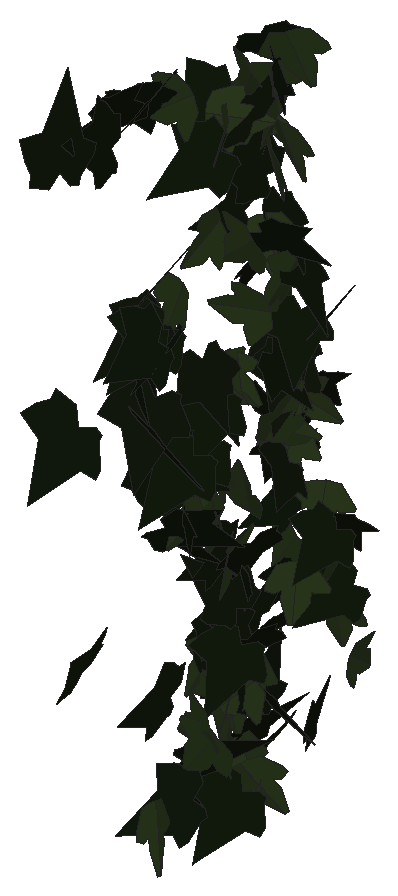
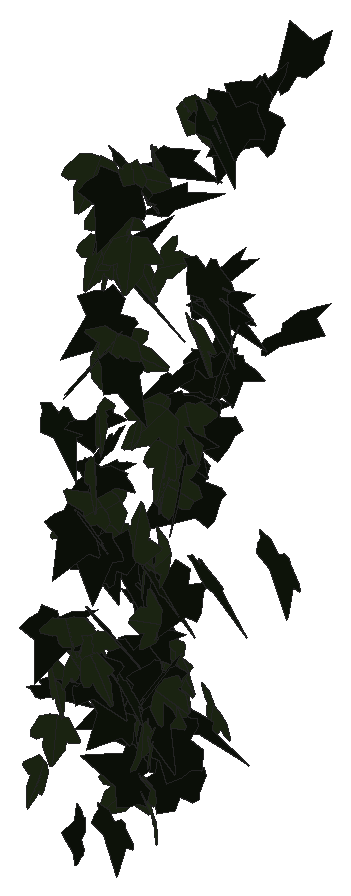
# SketchUp Ruby script. Lengths in inches.
U = 1.inch
M = Sketchup.active_model
def pt(a) = Geom::Point3d.new(a.map { |v| v * U })
def face(e, loops, mat)
  f = e.add_face(loops[0].map { |a| pt(a) })
  loops[1..].each { |l| e.add_face(l.map { |a| pt(a) }).erase! }
  f.material = f.back_material = mat if mat
  f
end
# faces: each face lists its corners as indices into pts; further lists are holes
def faces(e, pts, list, mat = nil) = list.each { |f| face(e, (f[0].is_a?(Array) ? f : [f]).map { |l| l.map { |i| pts[i] } }, mat) }
# xy, xz, yz: faces in a plane at the given z, y or x. An outline is a flat list of corners, or four numbers for a rectangle; further outlines are holes
def ring(l) = l.size == 4 ? [[l[0], l[1]], [l[2], l[1]], [l[2], l[3]], [l[0], l[3]]] : l.each_slice(2).to_a
def flat(e, list, mat, &to3) = list.each { |f| face(e, (f[0].is_a?(Array) ? f : [f]).map { |l| ring(l).map { |u, v| to3.(u, v) } }, mat) }
def xy(e, z, list, mat = nil) = flat(e, list, mat) { |x, y| [x, y, z] }
def xz(e, y, list, mat = nil) = flat(e, list, mat) { |x, z| [x, y, z] }
def yz(e, x, list, mat = nil) = flat(e, list, mat) { |y, z| [x, y, z] }
def lines(e, pts, list) = list.each { |a, b| e.add_line(pt(pts[a]), pt(pts[b])) }
# prism: a flat outline (further loops are holes) pulled along v
def prism(e, loops, v, mat = nil)
  f = face(e, loops, mat); d = Geom::Vector3d.new(v.map { |x| x * U })
  f.pushpull(f.normal.samedirection?(d) ? d.length : -d.length)
end
def box(e, o, s, mat = nil) = prism(e, [[o, [o[0] + s[0], o[1], o[2]], [o[0] + s[0], o[1] + s[1], o[2]], [o[0], o[1] + s[1], o[2]]]], [0, 0, s[2]], mat)
def at(x, y, z, deg = 0) = Geom::Transformation.translation(pt([x, y, z])) * Geom::Transformation.rotation(ORIGIN, Z_AXIS, deg.degrees)
def axes(o, x, y, z) = Geom::Transformation.new([*x, 0, *y, 0, *z, 0, *pt(o).to_a, 1])
def part(name) = M.definitions.add(name)
# library, detail: a bought-in or finely detailed component or shape, given as its bounding box
def library(name, o, s) = part(name).tap { |d| box(d.entities, o, s) }
def detail(e, o, s) = box(e.add_group.entities, o, s)
def put(e, d, t, mat = nil) = e.add_instance(d, t).tap { |i| i.material = mat if mat }
def group(e, t, mat = nil) = e.add_group.tap { |g| g.transformation = t; g.material = mat if mat }.entities
root = M.entities
M.materials.add("efeu1").color = [18, 25, 13]
M.materials.add("efeu2").color = [43, 57, 29]
c1 = part("ivyleaf_10")
p = [[0,0.5,-0.03],[-0.0625,2.02,-0.43],[-0.19,2.01,-0.46],[-0.54,1.05,-0.29],[-0.52,0.625,-0.18],[-0.83,0.76,-0.28],
  [-1.16,0.64,-0.33],[-1.15,0.33,-0.24],[-0.77,-0.39,0.02],[-0.3,-0.51,0.16],[0.04,-0.48,0.23],[-0.02,2.01,-0.4375],
  [-0.06,2.01,-0.43],[0.04,-0.49,0.23],[0.67,-0.49,0.14],[1.38,0.36,-0.2],[1.375,0.51,-0.24],[0.81,0.65,-0.19],
  [0.62,0.59,-0.15],[0.6,1.09,-0.28],[0.5,1.23,-0.31]]
faces(c1.entities,p,[[0,1,2,3,4,5,6,7,8,9,10],[11,12,0,13,14,15,16,17,18,19,20]],"efeu2")
c2 = part("ivyleaf_9")
p = [[1.54,2.16,1.25],[1.36,2.04,1.19],[-0.21,0.99,0.68],[-0.71,1.11,0.82],[-0.85,0.86,0.67],[-0.8,0.17,0.21],
  [-0.9,-0.01,0.1],[-0.67,-0.16,-0.02],[-0.08,-0.08,-0.05],[-0.03,-0.6,-0.4],[0.65,-0.88,-0.66],[0.83,-0.6,-0.49],
  [1.29,-0.42,-0.43],[1.8125,-0.07,-0.26],[1.21,0.44,0.15]]
faces(c2.entities,p,[[0,1,2,3,4,5,6,7,8,9,10,11,12,13,14]],"efeu1")
put(root,c1,axes([501.72,128.93,272.02],[-0.78096,-0.6795,-0.10689],[0.05982,0.09109,-1.03155],[0.73979,-0.72468,-0.02943]))
put(root,c2,axes([502.21,117.86,251.28],[-0.29268,0.97314,0.57352],[-0.16847,0.52899,-1.05055],[-1.19621,-0.3126,0.00763]))
put(root,c1,axes([501.68,126.66,248.28],[-0.09087,-0.69391,0.75827],[0.12672,-0.76299,-0.68304],[1.02001,0.03297,0.15241]))
put(root,c2,axes([502.08,129.67,242.97],[-0.12007,0.83731,0.36079],[-0.10194,0.33692,-0.87717],[-0.97351,-0.13855,0.04735]))
put(root,c2,axes([502.22,126.26,272.94],[-0.68822,-0.27679,0.78402],[-0.61332,-0.52516,-0.69977],[0.61326,-0.83583,0.18003]))
put(root,c2,axes([501.44,125.36,253.35],[1.1608,0.21664,-0.27086],[-0.31452,0.14824,-1.12166],[-0.18691,1.09594,0.20526]))
put(root,c2,axes([502.32,126.64,247.25],[0.30514,0.22931,-0.9611],[-0.97083,-0.2536,-0.35127],[-0.33906,0.9325,0.14081]))
put(root,c1,axes([501.35,127.875,242.7],[-0.3025,0.00297,-0.93347],[0.46003,-0.82719,-0.14109],[-0.85327,-0.44702,0.25487]))
put(root,c1,axes([502.36,130.77,251.37],[-0.76072,0.09915,0.57402],[-0.60564,-0.12345,-0.7212],[-0.00074,-0.8863,0.16467]))
put(root,c2,axes([502.51,130.46,253.66],[-0.94565,0.41354,0.12892],[-0.12249,0.04165,-1.03206],[-0.4155,-0.95349,0.01083]))
put(root,c2,axes([501.66,119.5,274.81],[0.56458,0.79306,0.80806],[0.4864,0.6335,-0.9876],[-1.09598,0.68968,-0.02204]))
put(root,c1,axes([502.04,126.88,251.94],[0.27281,-0.49023,0.87991],[-0.24877,0.81942,0.56531],[-1.02634,-0.32893,0.09686]))
put(root,c2,axes([501.3,130.58,256.63],[-0.01634,-0.24646,1.0091],[0.78003,-0.66939,-0.15086],[0.68598,0.75529,0.19558]))
put(root,c2,axes([502.65,128.3125,249.42],[-0.33388,0.68229,0.61589],[-0.33221,0.50902,-0.77692],[-0.91743,-0.43263,0.05719]))
put(root,c2,axes([502.13,121.05,275.42],[0.6466,0.91322,-0.19977],[-0.12195,-0.15565,-1.13562],[-1.00046,0.60919,0.00931]))
put(root,c2,axes([501.7,126.62,249.36],[0.51989,-0.80612,-0.39129],[-0.1805,0.34889,-0.9586],[0.8777,0.54925,0.03463]))
put(root,c2,axes([502.28,130.8,257.76],[0.64094,0.53886,-0.51639],[-0.41388,-0.31635,-0.83341],[-0.6745,0.70616,0.02069]))
put(root,c2,axes([501.85,126.65,249.34],[0.09255,-0.43655,-1.00064],[-0.15444,0.95164,-0.4623],[1.13058,0.16573,0.01876]))
put(root,c1,axes([502.3,127.27,245.49],[-0.11036,0.91847,-0.43534],[-0.04461,0.41658,0.96109],[1.0892,0.11013,-0.00474]))
put(root,c1,axes([502.49,130.73,261.33],[-0.69678,0.59318,0.37254],[-0.44044,0.07068,-0.8856],[-0.60506,-0.73455,0.21563]))
put(root,c1,axes([502.22,123.66,265.4],[0.98062,-0.57679,-0.12791],[-0.11605,0.06021,-1.11869],[0.62627,0.91429,-0.00702]))
put(root,c2,axes([502.7,121.59,275.1875],[-0.37673,1.046,0.02923],[-0.01204,0.0259,-1.14673],[-1.13002,-0.34899,0.00248]))
put(root,c2,axes([502.25,129.01,248.27],[0.40688,0.66465,0.56286],[0.12667,0.54564,-0.78181],[-0.91699,0.37029,0.14175]))
put(root,c2,axes([502.9375,125.71,253.41],[-0.87145,0.63548,0.10554],[-0.08486,0.06424,-1.06818],[-0.68981,-0.81072,-0.00192]))
put(root,c1,axes([502.69,125.27,254.37],[0.29546,-0.21031,0.99562],[-0.61259,0.77661,0.34601],[-0.8633,-0.62305,0.09521]))
put(root,c2,axes([502.68,121.54,261.6875],[0.13142,-0.8987,0.78595],[0.02404,0.7614,0.93794],[-1.26792,-0.07871,0.09924]))
put(root,c2,axes([502.39,128.78,274.71],[0.60354,0.84814,-0.01727],[-0.00637,-0.016,-1.05631],[-0.91614,0.55885,-0.00403]))
put(root,c2,axes([502.75,131.06,258.8125],[-0.94972,0.23126,-0.22964],[0.23788,-0.03027,-0.94525],[-0.25032,-0.90616,-0.02703]))
put(root,c2,axes([502.91,121.4,265.32],[-1.1589,-0.1407,0.02537],[-0.02545,-0.00795,-1.12552],[0.15211,-1.0733,0.00501]))
put(root,c2,axes([502.44,117.17,262.4],[-0.51227,-1.08029,0.53888],[-0.21565,-0.47821,-1.227],[1.27589,-0.51457,0.00897]))
put(root,c2,axes([502.85,128.32,265.54],[-0.40997,0.86111,-0.42499],[0.15795,-0.38203,-0.97852],[-1.01722,-0.40638,0.01934]))
put(root,c2,axes([503.04,121.88,267.28],[-0.4821,1.07553,-0.04386],[-0.00007,-0.04568,-1.21093],[-1.16246,-0.44604,0.01826]))
put(root,c2,axes([502.82,130.18,250.71],[-0.08384,0.5825,-0.74236],[0.0297,-0.71455,-0.60954],[-0.99458,-0.07044,0.04437]))
put(root,c2,axes([502.61,131.37,242.76],[0.04801,-0.00313,0.90204],[0.2179,0.8447,-0.00759],[-0.91104,0.20187,0.04572]))
put(root,c1,axes([502.43,128.02,273.21],[-0.67854,0.77843,-0.17211],[0.10682,-0.13283,-1.04034],[-0.85283,-0.63599,0.00663]))
put(root,c2,axes([503.26,126.41,268.26],[-0.84821,0.56452,0.24472],[-0.24715,0.08392,-1.00373],[-0.61255,-0.81556,0.06611]))
put(root,c1,axes([502.58,126.25,247.27],[-1.09261,-0.41527,-0.15628],[0.1886,-0.03118,-1.13309],[0.43807,-1.0223,0.09804]))
put(root,c1,axes([502.38,128.18,271.125],[0.39667,0.94718,0.03913],[0.01781,0.03395,-1.05653],[-1.02361,0.36764,-0.00322]))
put(root,c2,axes([502.24,124.85,242.35],[0.77152,0.6545,0.4461],[-0.33554,-0.29584,1.00759],[0.77568,-0.77897,-0.00785]))
put(root,c1,axes([502.3125,126.85,245.67],[0.00305,0.02034,-1.06011],[0.27283,-0.98757,-0.01977],[-1.06677,-0.25251,-0.00809]))
put(root,c2,axes([502.74,118.9,274.18],[-0.1507,-0.14254,1.17854],[-0.49712,-1.0378,-0.19471],[1.1289,-0.47604,0.07159]))
put(root,c2,axes([502.86,115.69,274.72],[-0.51525,-0.72738,0.993],[0.66598,0.73298,0.90117],[-1.11218,0.7759,0.07959]))
put(root,c1,axes([502.89,123.36,260.6],[-0.1271,-1.05619,0.07366],[-0.00448,-0.0708,-1.10523],[1.14324,-0.1177,0.00385]))
put(root,c1,axes([502.875,128.75,273.29],[-0.82233,-0.65785,-0.09973],[0.0826,0.05815,-1.04647],[0.71322,-0.76523,0.00621]))
put(root,c2,axes([502.4,127.52,244.3],[0.0977,0.92451,-0.40102],[0.0265,0.38501,0.966],[1.08151,-0.09295,0.01255]))
put(root,c2,axes([503.1,129.39,256.82],[0.09782,0.81046,-0.50619],[-0.10808,-0.47799,-0.84711],[-1.01528,0.12897,0.04141]))
put(root,c2,axes([502.8,130.98,258.36],[0.52486,0.77685,0.19284],[0.11522,0.15197,-0.95294],[-0.85484,0.49746,-0.01003]))
put(root,c2,axes([503.72,125.37,251.48],[-0.20153,0.3281,0.95737],[-0.90014,0.43593,-0.33729],[-0.55111,-0.83199,0.20081]))
put(root,c2,axes([502.4,124.15,244.7],[0.17546,0.77238,-0.84602],[0.17513,0.79716,0.82084],[1.19876,-0.22951,0.00391]))
put(root,c1,axes([503.5,126.72,274.12],[-0.88327,0.27039,0.66885],[-0.65869,0.20404,-0.89583],[-0.36583,-1.02022,-0.0019]))
put(root,c2,axes([502.47,129.93,266.83],[0.40664,-0.8982,0.01344],[0.01251,-0.00916,-1.01286],[0.97008,0.37663,0.00743]))
put(root,c2,axes([502.61,129.93,260.92],[-0.52396,-0.62003,-0.67499],[0.58726,0.36983,-0.79557],[0.70368,-0.77031,0.16135]))
put(root,c1,axes([502.85,129.64,263.35],[0.35109,-0.97546,0.2369],[0.34439,-0.11869,-0.99911],[0.94289,0.40657,0.27671]))
put(root,c1,axes([503.08,131.4,251.75],[-0.16641,0.71349,-0.57631],[-0.12014,-0.57285,-0.73492],[-0.96826,-0.05155,0.19023]))
put(root,c1,axes([503.21,126.71,255.28],[-1.05007,0.19697,0.03456],[0.03125,-0.02454,1.03155],[0.21346,0.97255,0.01902]))
put(root,c1,axes([503.7,122.12,275.28],[0.73402,-0.19724,-0.85795],[-0.82942,0.30568,-0.73403],[0.38889,1.02422,0.05385]))
put(root,c1,axes([502.56,127.27,243.9],[0.84539,0.00314,0.6131],[0.63661,-0.01972,-0.81388],[0.0101,0.97973,-0.01835]))
put(root,c2,axes([503.76,125.78,253.02],[0.10141,0.08594,-1.01237],[-1.05528,-0.00627,-0.0986],[-0.01568,0.97793,0.08833]))
put(root,c2,axes([503.41,121.21,265.31],[-0.83727,-0.71043,0.23086],[-0.17764,-0.14907,-1.0936],[0.78398,-0.79251,-0.00125]))
put(root,c1,axes([502.87,125.61,261.54],[-0.69758,-0.41775,-0.69608],[0.68153,0.19729,-0.80141],[0.44109,-0.96551,0.13741]))
put(root,c1,axes([503.17,131.54,253.52],[0.82028,0.49041,-0.09924],[-0.07878,-0.06292,-0.94015],[-0.5338,0.7629,-0.01375]))
put(root,c2,axes([503.52,128.14,274.08],[0.51,-0.10683,-0.93608],[-0.87215,0.4113,-0.4914],[0.44454,0.9295,0.10986]))
put(root,c1,axes([503.8,125.98,247.63],[0.81202,-0.01274,-0.67385],[-0.69618,0.0875,-0.77973],[0.07208,0.98867,0.06033]))
put(root,c2,axes([503.21,129.58,260.22],[-0.33939,-1.01454,0.0589],[0.01675,-0.06767,-1.06916],[1.01611,-0.33775,0.03729]))
put(root,c2,axes([503.32,120.91,262.28],[-0.97572,-0.66022,-0.48489],[0.40607,0.27571,-1.16374],[0.77272,-0.97856,-0.00073]))
put(root,c2,axes([504.18,122.05,244.44],[-1.20392,0.17857,0.30785],[-0.31574,0.04639,-1.17412],[-0.19926,-1.15244,0.00044]))
put(root,c1,axes([503.33,124.94,261.65],[-0.09444,0.79519,0.72775],[-0.05462,0.72607,-0.80044],[-1.07655,-0.10659,-0.02323]))
put(root,c2,axes([503.82,127.08,269.84],[-0.19751,0.07639,1.06889],[-0.8386,-0.69658,-0.08985],[0.73189,-0.77753,0.1855]))
put(root,c1,axes([503.02,128.29,266.61],[0.9831,0.319,0.35597],[0.34955,0.11136,-1.00313],[-0.3649,0.9661,-0.00191]))
put(root,c1,axes([503.41,129.23,257.11],[0.94753,0.33113,-0.15832],[-0.15166,-0.05904,-0.97524],[-0.36321,0.88849,-0.0058]))
put(root,c1,axes([503.4,124.88,246.18],[-0.54743,0.8672,-0.0376],[0.01982,-0.03116,-1.04465],[-0.93718,-0.50721,-0.00013]))
put(root,c1,axes([503.62,131.95,248.43],[-0.93335,-0.19237,0.04711],[-0.0445,-0.02337,-0.92067],[0.20875,-0.86508,0.0144]))
put(root,c2,axes([503.03,121.25,259.45],[0.25769,-0.09773,-1.22069],[-0.08279,1.19376,-0.11957],[1.26933,0.0977,0.24002]))
put(root,c2,axes([503.75,126.2,249.54],[0.12437,0.94431,-0.26799],[-0.03234,-0.25594,-0.98936],[-1.05665,0.11898,-0.00127]))
put(root,c2,axes([503.77,123.47,259.38],[-1.04224,-0.56009,-0.15295],[0.11804,0.10452,-1.15985],[0.61416,-0.97057,-0.03664]))
put(root,c2,axes([504.22,120.2,264.83],[-0.51275,1.03756,0.20388],[-0.12785,0.16129,-1.18594],[-1.13321,-0.48767,0.04155]))
put(root,c1,axes([503.6,124.32,268.47],[0.10217,0.3736,-1.04423],[-0.21587,-0.98412,-0.40042],[-1.13671,0.22047,-0.01781]))
put(root,c1,axes([503.71,124.08,258.64],[-1.0243,0.45629,0.11146],[-0.10397,0.04711,-1.09458],[-0.49541,-0.9533,-0.00074]))
put(root,c1,axes([503.8125,123.51,256.77],[-0.26663,-0.61891,0.87573],[-0.07577,-0.85346,-0.67378],[1.12609,-0.20397,0.16202]))
put(root,c1,axes([503.73,131.78,250.82],[0.25255,-0.86865,-0.07681],[-0.03132,0.06868,-0.9355],[0.94101,0.23542,-0.01052]))
put(root,c2,axes([503.86,122.37,257.39],[0.42845,-0.25651,-1.02312],[-0.92131,0.49049,-0.49077],[0.59732,0.94053,-0.0231]))
put(root,c1,axes([503.1,129.9375,258.5625],[0.54841,0.20725,0.88486],[0.55429,0.74273,-0.51749],[-0.72021,0.72944,0.27552]))
put(root,c1,axes([503.53,125.49,253.83],[-0.26729,0.59919,-0.80041],[0.06646,-0.78284,-0.65443],[-1.0513,-0.20183,0.16213]))
put(root,c1,axes([503.24,128.3125,271.52],[0.00388,0.0197,1.06145],[0.69067,-0.79557,0.01363],[0.85932,0.63934,-0.01574]))
put(root,c1,axes([503.99,122.37,258.03],[-0.13601,0.21203,1.10607],[-0.53144,0.94294,-0.25611],[-1.0437,-0.50776,-0.01373]))
put(root,c1,axes([504.5,125.78,264.59],[0.21446,0.04379,-1.04068],[-1.07198,0.14535,-0.19823],[0.145,1.00976,0.07367]))
put(root,c1,axes([503.38,126.79,243.33],[-0.85887,-0.24834,-0.6251],[0.62949,0.14897,-0.86604],[0.31154,-0.98565,0.02661]))
put(root,c1,axes([503.39,128.3,257.99],[-0.35284,-0.33743,-0.89319],[0.64467,0.61749,-0.48846],[0.75997,-0.68047,-0.00034]))
put(root,c1,axes([504.57,122.55,247.47],[-0.45503,0.04623,0.99267],[-1.0181,0.15088,-0.44036],[-0.16917,-1.03238,-0.01991]))
put(root,c2,axes([503.39,123.95,262.68],[0.31021,-0.95965,-0.5692],[-0.14841,0.53007,-1.04162],[1.18386,0.31791,0.01857]))
put(root,c2,axes([503.57,128.0625,261.23],[0.52717,-0.52357,-0.69228],[-0.39854,0.56004,-0.73954],[0.82324,0.60639,0.08529]))
put(root,c1,axes([503.68,127.91,258.1],[-0.05884,-0.91706,0.48775],[0.02776,0.46829,0.95542],[-1.11208,0.06021,-0.00196]))
put(root,c1,axes([503.78,128.56,270.98],[-1.016,0.35149,-0.14254],[0.14658,-0.02825,-1.0442],[-0.38017,-0.95025,-0.02168]))
put(root,c2,axes([503.4,121.78,256.33],[0.92733,0.68329,0.54176],[0.43496,0.33048,-1.14121],[-0.8197,0.94838,0.00734]))
put(root,c2,axes([503.82,126.8,246.65],[-0.17014,-0.50171,0.8615],[0.62665,0.62305,0.50721],[-0.83742,0.56817,0.20452]))
put(root,c1,axes([504.11,132.37,246.15],[0.06777,0.49284,0.7562],[-0.40657,0.67372,-0.44113],[-0.85714,-0.2806,0.26903]))
put(root,c2,axes([503.95,124.02,261.1875],[-0.62245,-0.8518,-0.01068],[0.00758,0.00766,-1.06959],[0.91998,-0.57638,0.00158]))
put(root,c1,axes([503.64,126.56,248.24],[1.01168,-0.09174,0.29659],[0.31076,0.01503,-0.97794],[0.09003,0.97907,0.0428]))
put(root,c2,axes([503.8125,129.36,262.65],[-0.36836,-0.91749,-0.19117],[0.06311,0.17438,-1.01797],[1.00861,-0.34599,-0.00612]))
put(root,c1,axes([504.34,123.21,257.6],[-0.60158,0.58799,0.65844],[-0.48853,0.44336,-0.84211],[-0.79507,-0.71731,0.01923]))
put(root,c2,axes([504.1,125.23,249.81],[-0.71305,-0.78739,0.01187],[-0.00372,-0.012,-1.06865],[0.85046,-0.66022,0.00527]))
put(root,c2,axes([504.79,125.12,273.375],[-0.38637,0.82498,0.63675],[-0.49344,0.45333,-0.88675],[-0.9179,-0.59095,0.20867]))
put(root,c2,axes([504.08,120.09,265.52],[-0.35993,-0.69205,0.90842],[-0.34582,-0.8138,-0.7976],[1.15281,-0.46019,0.04436]))
put(root,c1,axes([504.21,127.2,270.71],[-0.8018,0.70772,0.23513],[-0.19347,0.13602,-1.06916],[-0.72022,-0.82442,0.02544]))
put(root,c2,axes([504.38,125.55,254.27],[-0.04767,0.95541,-0.30981],[0.04555,-0.29614,-0.99429],[-1.07988,-0.05467,-0.02827]))
put(root,c1,axes([503.26,125.11,273.15],[0.10485,-0.30463,-1.00732],[1.09243,0.11356,0.0683],[0.09529,-0.96678,0.32543]))
put(root,c1,axes([504.03,128.58,275.12],[-0.96406,-0.45281,-0.30173],[0.28999,0.09185,-1.06441],[0.46042,-1.00599,0.03863]))
put(root,c1,axes([503.98,128.86,251.35],[0.81974,0.55403,-0.04832],[-0.03649,-0.03253,-0.97728],[-0.59935,0.75974,-0.0066]))
put(root,c2,axes([504.53,131.5,249.9],[-0.86119,-0.34755,0.26642],[-0.22773,-0.15601,-0.90274],[0.40691,-0.82288,0.05863]))
put(root,c1,axes([503.61,120.5625,244.21],[0.8662,-0.32864,0.67045],[0.64305,-0.24713,-0.90142],[0.44408,0.99889,-0.00243]))
put(root,c2,axes([503.27,120.48,261.26],[0.89727,-0.57473,0.48007],[0.41306,-0.2585,-1.05062],[0.68059,0.9146,0.00473]))
put(root,c2,axes([504.11,131.04,252.93],[0.77889,0.54112,-0.19509],[-0.23216,-0.02384,-0.93099],[-0.57331,0.74481,0.11194]))
put(root,c1,axes([504.81,122.59,246.96],[-0.89962,-0.04425,0.69478],[-0.70738,-0.16721,-0.86086],[0.14991,-1.05461,0.10734]))
put(root,c1,axes([504.39,123.89,273.47],[0.43411,-0.79143,-0.55573],[-0.19103,0.50803,-0.9209],[1.01348,0.43475,0.06446]))
put(root,c2,axes([504.7,123.13,272.8125],[-0.8817,-0.51672,0.45535],[-0.41545,-0.19093,-1.02112],[0.54931,-0.9738,-0.04141]))
put(root,c2,axes([504.4,124.88,243.55],[-0.81271,-0.78954,0.1656],[-0.09698,-0.13432,-1.13398],[0.86445,-0.75736,0.02847]))
put(root,c1,axes([504.1,128.17,265.16],[0.05886,-0.46691,0.95017],[0.31678,-0.86964,-0.48041],[1.06186,0.28532,0.09065]))
put(root,c2,axes([503.83,127.22,267.13],[0.95144,0.43116,0.29051],[0.27165,0.10427,-1.04445],[-0.44329,0.98932,-0.01653]))
put(root,c2,axes([504.61,121.57,259.95],[-1.00146,-0.63746,0.04647],[-0.02528,-0.04481,-1.17],[0.68968,-0.92727,0.02459]))
put(root,c2,axes([505.1,119.56,250.39],[-0.91981,0.77257,0.15062],[-0.12171,0.09131,-1.19584],[-0.84013,-0.85906,0.00834]))
put(root,c2,axes([504.5,130.54,252.76],[-0.59899,-0.71128,0.30687],[-0.08063,-0.31225,-0.92876],[0.82774,-0.54513,0.13159]))
put(root,c2,axes([504.875,130.05,262.86],[-0.34206,0.91809,0.02878],[-0.00772,0.02681,-1.01003],[-0.99195,-0.3168,-0.00206]))
put(root,c2,axes([504.1,128.23,256.61],[-0.07235,-0.75131,0.5887],[0.10205,-0.56999,-0.77517],[1.0108,0.00377,0.1204]))
put(root,c2,axes([503.75,126.78,247.17],[0.9804,-0.34692,0.20095],[0.20103,-0.05414,-1.01055],[0.37883,0.92654,0.01619]))
put(root,c1,axes([505.18,124.43,268.37],[-0.71302,-0.02073,0.83202],[-0.86426,0.006,-0.68664],[0.00925,-1.03724,-0.0206]))
put(root,c2,axes([503.93,129.16,265.14],[0.46673,-0.98535,-0.02273],[0.04155,0.0448,-1.08882],[0.98474,0.46513,0.05671]))
